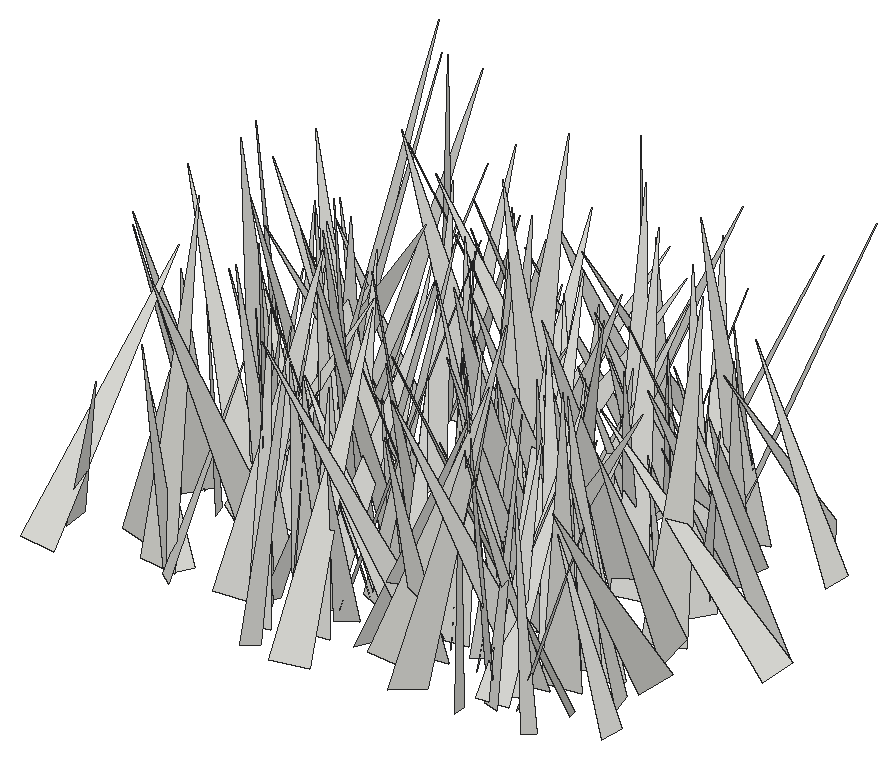
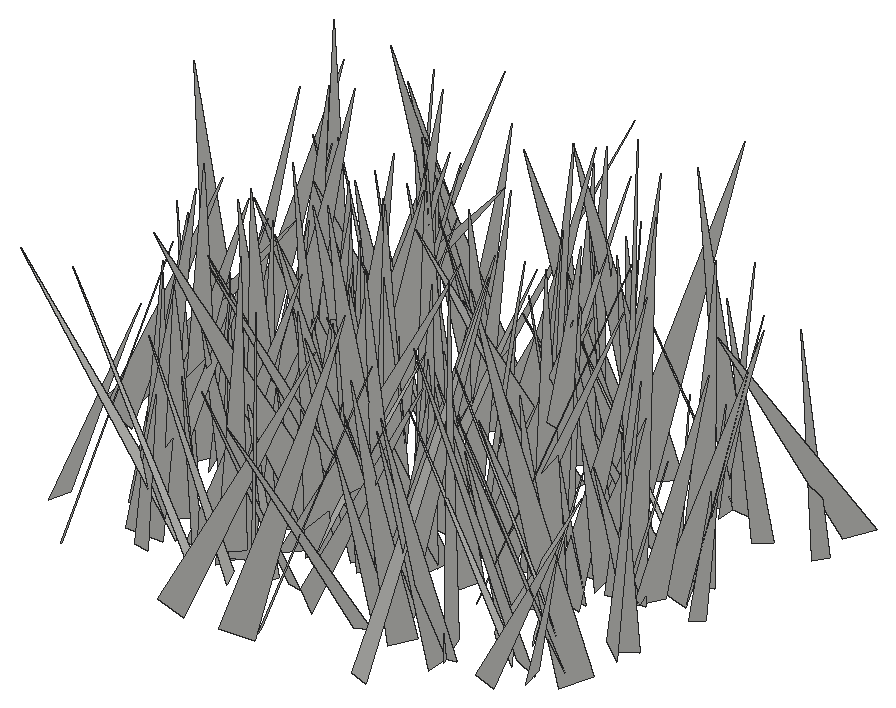
# SketchUp Ruby script. Lengths in inches.
U = 1.inch
M = Sketchup.active_model
def pt(a) = Geom::Point3d.new(a.map { |v| v * U })
def face(e, loops, mat)
  f = e.add_face(loops[0].map { |a| pt(a) })
  loops[1..].each { |l| e.add_face(l.map { |a| pt(a) }).erase! }
  f.material = f.back_material = mat if mat
  f
end
# faces: each face lists its corners as indices into pts; further lists are holes
def faces(e, pts, list, mat = nil) = list.each { |f| face(e, (f[0].is_a?(Array) ? f : [f]).map { |l| l.map { |i| pts[i] } }, mat) }
# xy, xz, yz: faces in a plane at the given z, y or x. An outline is a flat list of corners, or four numbers for a rectangle; further outlines are holes
def ring(l) = l.size == 4 ? [[l[0], l[1]], [l[2], l[1]], [l[2], l[3]], [l[0], l[3]]] : l.each_slice(2).to_a
def flat(e, list, mat, &to3) = list.each { |f| face(e, (f[0].is_a?(Array) ? f : [f]).map { |l| ring(l).map { |u, v| to3.(u, v) } }, mat) }
def xy(e, z, list, mat = nil) = flat(e, list, mat) { |x, y| [x, y, z] }
def xz(e, y, list, mat = nil) = flat(e, list, mat) { |x, z| [x, y, z] }
def yz(e, x, list, mat = nil) = flat(e, list, mat) { |y, z| [x, y, z] }
def lines(e, pts, list) = list.each { |a, b| e.add_line(pt(pts[a]), pt(pts[b])) }
# prism: a flat outline (further loops are holes) pulled along v
def prism(e, loops, v, mat = nil)
  f = face(e, loops, mat); d = Geom::Vector3d.new(v.map { |x| x * U })
  f.pushpull(f.normal.samedirection?(d) ? d.length : -d.length)
end
def box(e, o, s, mat = nil) = prism(e, [[o, [o[0] + s[0], o[1], o[2]], [o[0] + s[0], o[1] + s[1], o[2]], [o[0], o[1] + s[1], o[2]]]], [0, 0, s[2]], mat)
def at(x, y, z, deg = 0) = Geom::Transformation.translation(pt([x, y, z])) * Geom::Transformation.rotation(ORIGIN, Z_AXIS, deg.degrees)
def axes(o, x, y, z) = Geom::Transformation.new([*x, 0, *y, 0, *z, 0, *pt(o).to_a, 1])
def part(name) = M.definitions.add(name)
# library, detail: a bought-in or finely detailed component or shape, given as its bounding box
def library(name, o, s) = part(name).tap { |d| box(d.entities, o, s) }
def detail(e, o, s) = box(e.add_group.entities, o, s)
def put(e, d, t, mat = nil) = e.add_instance(d, t).tap { |i| i.material = mat if mat }
def group(e, t, mat = nil) = e.add_group.tap { |g| g.transformation = t; g.material = mat if mat }.entities
root = M.entities
c1 = part("fur_instance\#9")
p = [[0.8125,0,1.79],[0.67,-0.02,1.48],[0,-0.11,0],[0,0.11,0]]
faces(c1.entities,p,[[0,1,2,3]])
put(root,c1,axes([127.42,270.56,-27.1],[0.8568,-5.86099,0.80486],[-5.91149,-0.87995,-0.11477],[-0.231,0.77949,5.92218]))
put(root,c1,axes([121.75,270.07,-27.1],[1.49133,-6.04191,1.54576],[-6.23212,-1.50337,0.13646],[-0.23383,1.53405,6.22175]))
put(root,c1,axes([127.07,271.05,-27.1],[-7.35388,-1.92649,0.06127],[-1.88282,7.23164,1.39751],[0.41243,-1.33667,7.47248]))
put(root,c1,axes([123.36,266.85,-27.1],[-3.83392,6.10516,1.11787],[5.9137,3.99214,-1.52073],[1.88436,-0.10697,7.04694]))
put(root,c1,axes([114.97,270.12,-27.1],[-4.71927,-1.33587,1.95814],[-1.09743,5.09822,0.83318],[2.10107,-0.33763,4.83341]))
put(root,c1,axes([122.98,270.82,-27.1],[2.32528,-3.90872,0.2043],[-3.90658,-2.33236,-0.15975],[-0.24182,0.09371,4.54527]))
put(root,c1,axes([130.97,271.93,-27.1],[-7.04471,-1.4589,1.32068],[-0.96261,6.83613,2.41686],[1.71638,-2.15394,6.77607]))
put(root,c1,axes([130.64,268.0625,-27.1],[-5.01766,-1.40088,1.70753],[-1.93126,4.83928,-1.7049],[1.07162,2.16194,4.92267]))
put(root,c1,axes([109.97,270.61,-27.1],[4.41728,-0.60705,0.29796],[-0.51929,-4.30631,-1.07505],[-0.43316,-1.02804,4.32726]))
put(root,c1,axes([121.25,267.11,-27.1],[-5.97598,0.81352,1.54005],[0.17172,5.75229,-2.37225],[1.73323,2.235,5.54496]))
put(root,c1,axes([121.75,270.68,-27.1],[4.45698,-3.93649,1.376],[-3.92382,-4.64074,-0.56675],[-1.41173,0.47074,5.91941]))
put(root,c1,axes([128.1,268.14,-27.1],[7.25129,-2.23194,2.73946],[-2.93898,-7.28136,1.84704],[-1.96177,2.6585,7.35875]))
put(root,c1,axes([121.08,269.83,-27.1],[4.15437,2.45212,1.76514],[2.75663,-4.30471,-0.50784],[-1.23677,-1.35794,4.79727]))
put(root,c1,axes([126.07,269.39,-27.1],[3.27115,-5.93629,2.22387],[-6.24966,-2.60094,2.25],[1.06155,2.98013,6.39355]))
put(root,c1,axes([118,272.57,-27.1],[3.07442,-7.15508,0.96712],[-6.88437,-3.22185,-1.95131],[-2.1762,0.08396,7.5392]))
put(root,c1,axes([122.84,269.21,-27.1],[-0.37436,4.96388,1.61425],[5.21969,0.34743,0.14211],[-0.02763,-1.62026,4.97594]))
put(root,c1,axes([132.09,270.02,-27.1],[4.65437,1.55789,0.49043],[1.62302,-4.57734,-0.86283],[-0.1826,-0.97553,4.83174]))
put(root,c1,axes([136.32,270.28,-27.1],[-4.20728,0.83557,0.99678],[1.00115,4.23485,0.67581],[0.83033,-0.87227,4.23588]))
put(root,c1,axes([130.74,269.85,-27.1],[3.92843,5.06138,3.38638],[5.5366,-4.64662,0.52215],[-2.53598,-2.30413,6.38572]))
put(root,c1,axes([120.65,268.35,-27.1],[0.64289,6.12986,1.03372],[6.0316,-0.86662,1.38779],[-1.50455,-0.85491,6.00521]))
put(root,c1,axes([133.84,268.3,-27.1],[-4.92435,-0.05312,0.24709],[-0.15186,4.47527,-2.06445],[0.20202,2.06935,4.47102]))
put(root,c1,axes([119.71,270.26,-27.1],[4.16125,-1.09144,0.28201],[-1.11074,-4.15389,0.31328],[-0.19241,0.37504,4.29058]))
put(root,c1,axes([112.49,270.96,-27.1],[0.76926,-4.66703,1.07076],[-4.59745,-0.41678,1.48633],[1.33832,1.25083,4.49041]))
put(root,c1,axes([126.06,270.8,-27.1],[-4.18794,0.93567,0.33129],[0.9893,4.05153,1.06324],[0.08071,-1.11073,4.15738]))
put(root,c1,axes([124.67,269.99,-27.1],[6.16079,-1.33707,0.34037],[-1.37023,-6.11166,0.79308],[-0.16154,0.84778,6.25413]))
put(root,c1,axes([132.01,271.26,-27.1],[-1.08629,-5.09453,1.21583],[-5.17343,0.84989,-1.06105],[-0.81738,1.39139,5.09985]))
put(root,c1,axes([115.7,270.01,-27.1],[-3.05082,2.35934,0.28628],[2.37608,3.01778,0.45074],[-0.05159,-0.53147,3.83025]))
put(root,c1,axes([114.69,269.6875,-27.1],[0.76042,7.54721,2.45249],[7.93568,-0.724,-0.23253],[-0.00259,-2.46349,7.58186]))
put(root,c1,axes([135.22,274.29,-27.1],[5.40671,-4.03304,0.21931],[-3.53675,-4.90438,-2.9974],[-1.95061,-2.2864,6.04264]))
put(root,c1,axes([119.75,270.36,-27.1],[4.32475,3.25099,2.86901],[3.37923,-5.06616,0.64681],[-2.71679,-1.12634,5.37159]))
put(root,c1,axes([115.56,269.07,-27.1],[2.99735,3.72962,0.28981],[3.68324,-3.00724,0.60693],[-0.65404,0.15682,4.74613]))
put(root,c1,axes([132.59,271.86,-27.1],[2.16747,-6.96935,1.82134],[-7.20329,-2.08612,0.58967],[0.04123,1.91397,7.27476]))
put(root,c1,axes([131.39,269.05,-27.1],[2.56304,5.03632,1.18387],[4.82189,-2.80423,1.49027],[-1.87495,-0.32715,5.45094]))
put(root,c1,axes([118.48,269.61,-27.1],[-2.56408,6.91655,2.55207],[6.94878,3.17004,-1.60986],[2.46298,-1.74312,7.19872]))
put(root,c1,axes([134.1875,270.53,-27.1],[-5.38862,-5.55187,0.24968],[-4.68183,4.34761,-4.37054],[-2.99434,3.19341,6.38427]))
put(root,c1,axes([118.8125,271.9,-27.1],[-6.63003,0.58928,2.6026],[0.94805,7.03587,0.82207],[2.49439,-1.10786,6.6052]))
put(root,c1,axes([131.35,269.95,-27.1],[-4.05743,3.11883,1.27429],[2.94276,4.25195,-1.03673],[1.64046,0.08657,5.0115]))
put(root,c1,axes([110.04,268.16,-27.1],[-2.9172,5.75801,0.16061],[5.28877,2.74872,-2.48273],[2.2824,0.99014,5.95825]))
put(root,c1,axes([126.52,270.12,-27.1],[-2.91757,4.706,0.99504],[4.75363,2.9987,-0.24403],[0.73452,-0.71423,5.53165]))
put(root,c1,axes([129.02,271.27,-27.1],[3.30079,2.00098,0.99665],[2.11543,-3.37049,-0.23912],[-0.72261,-0.72685,3.85253]))
put(root,c1,axes([122.03,273.26,-27.1],[-4.79453,-5.10071,1.01007],[-5.15614,4.84133,-0.02673],[0.67211,0.75447,7.00029]))
put(root,c1,axes([128.05,273.51,-27.1],[5.66121,2.03663,0.41958],[1.99596,-4.98096,-2.75306],[0.58316,-2.72311,5.34956]))
put(root,c1,axes([135.13,272.32,-27.1],[-4.98874,-1.77944,1.14235],[-1.81158,5.1064,0.04294],[1.09068,0.3424,5.29642]))
put(root,c1,axes([131.25,269.32,-27.1],[-3.49002,4.97532,0.38419],[4.70613,3.43753,-1.76559],[1.65943,0.71499,5.81522]))
put(root,c1,axes([116.8,273.88,-27.1],[-4.19902,-6.23031,2.61813],[-6.01537,4.8505,1.89504],[3.08005,0.97931,7.27031]))
put(root,c1,axes([127.11,272.03,-27.1],[-1.46748,5.77462,2.34569],[6.13429,1.76496,-0.50731],[1.10405,-2.13089,5.93652]))
put(root,c1,axes([126.41,272.37,-27.1],[5.41159,0.09186,1.28906],[0.07062,-5.56242,0.09991],[-1.29039,0.08081,5.41145]))
put(root,c1,axes([132.98,273.75,-27.1],[2.11565,-6.08651,1.80009],[-6.2822,-2.27872,-0.32139],[-0.90548,1.58863,6.43571]))
put(root,c1,axes([116.19,273.82,-27.1],[5.48101,-1.25937,0.85366],[-1.15676,-5.52263,-0.72019],[-0.98826,-0.52035,5.57753]))
put(root,c1,axes([116.03,272.39,-27.1],[3.45283,2.51437,0.03768],[2.48973,-3.40925,-0.65094],[0.3531,-0.54815,4.22141]))
put(root,c1,axes([123.1,273.23,-27.1],[-4.21656,2.08304,0.19454],[2.06998,4.09043,1.06765],[-0.30342,-1.04195,4.58024]))
put(root,c1,axes([128.22,275.07,-27.1],[-3.59271,-3.52154,0.36411],[-3.38524,3.56898,1.11534],[1.03633,-0.55007,4.90559]))
put(root,c1,axes([133.88,273.48,-27.1],[1.42768,-3.34431,1.65268],[-3.54003,-1.77266,-0.52903],[-1.17641,1.27565,3.59761]))
put(root,c1,axes([123.36,275.24,-27.1],[-0.67207,-6.04885,0.74296],[-6.03248,0.76649,0.78356],[0.86591,0.6451,6.03542]))
put(root,c1,axes([129.29,274.77,-27.1],[-0.74587,-6.40704,1.23448],[-6.45249,0.53969,-1.09751],[-0.96927,1.33753,6.35625]))
put(root,c1,axes([112.27,275.28,-27.1],[4.76035,-4.27512,0.72339],[-4.20428,-4.81383,-0.78223],[-1.06017,-0.10597,6.35025]))
put(root,c1,axes([134.24,276.65,-27.1],[6.25747,-1.85529,1.59771],[-1.00282,-5.94215,-2.97253],[-2.23363,-2.52972,5.81052]))
put(root,c1,axes([127.14,271.94,-27.1],[5.31118,5.11176,2.74997],[4.78098,-5.96627,1.85658],[-3.29161,-0.41778,7.13385]))
put(root,c1,axes([129.2,273.22,-27.1],[-7.32876,-0.97242,0.83606],[-1.07916,7.29688,-0.97277],[0.69283,1.07947,7.32872]))
put(root,c1,axes([121.81,275.6,-27.1],[-2.25691,-7.5793,1.44794],[-7.71352,2.17504,-0.63772],[-0.20948,1.56823,7.88243]))
put(root,c1,axes([125.21,274.68,-27.1],[-3.55918,-3.90599,0.48478],[-3.91702,3.45103,-0.95229],[-0.38568,0.99656,5.19785]))
put(root,c1,axes([128.62,271.69,-27.1],[1.86893,4.92203,0.04113],[4.36091,-1.67616,2.42774],[-2.28266,0.8277,4.67176]))
put(root,c1,axes([124.77,275.62,-27.1],[4.05285,-0.43746,0.41546],[-0.3233,-3.95717,-1.01285],[-0.50937,-0.96903,3.94856]))
put(root,c1,axes([122.45,274.5,-27.1],[0.90627,3.33198,1.59944],[3.57947,-1.20149,0.47479],[-0.9207,-1.39138,3.42023]))
put(root,c1,axes([112.03,276.02,-27.1],[-5.14482,-3.13912,1.24988],[-3.04737,5.29445,0.7535],[1.4594,-0.01101,5.97959]))
put(root,c1,axes([113.89,274.38,-27.1],[-3.72029,-1.54775,1.40082],[-1.82397,3.80239,-0.64288],[1.01535,1.15959,3.97778]))
put(root,c1,axes([130.78,273.8,-27.1],[-2.14866,5.91991,1.32548],[6.06222,2.04254,0.70466],[-0.22751,-1.48381,6.25824]))
put(root,c1,axes([122.1875,271.52,-27.1],[6.2923,4.31715,0.79405],[3.75537,-6.01297,2.93303],[-2.27277,2.01685,7.04472]))
put(root,c1,axes([118.12,277.77,-27.1],[-1.88375,-7.99896,1.23534],[-7.80751,2.13018,1.88761],[2.13359,0.73274,7.99805]))
put(root,c1,axes([124.57,275.87,-27.1],[4.01557,-5.25956,2.05629],[-5.53772,-4.16187,0.169],[-1.10676,1.74125,6.61508]))
put(root,c1,axes([122.62,272.67,-27.1],[3.92721,6.27569,0.86047],[6.07775,-4.01843,1.56873],[-1.78486,0.12492,7.23508]))
put(root,c1,axes([125.4375,278.36,-27.1],[4.78768,-6.87101,0.53821],[-6.76798,-4.81092,-1.21319],[-1.30189,-0.25808,8.28619]))
put(root,c1,axes([112.44,276.5,-27.1],[-0.64276,-5.9949,1.38637],[-6.03632,0.34404,-1.31091],[-1.1932,1.48889,5.88502]))
put(root,c1,axes([120.71,272.51,-27.1],[-4.56425,4.1816,0.8559],[3.58274,4.43445,-2.55936],[2.31998,1.37862,5.63629]))
put(root,c1,axes([114.54,274.4,-27.1],[2.28513,5.39499,0.34939],[5.12885,-2.04337,-1.99232],[1.70965,-1.08097,5.50984]))
put(root,c1,axes([110.66,277.23,-27.1],[4.01864,-1.00258,0.99057],[-0.63294,-3.95809,-1.43832],[-1.25928,-1.21004,3.88405]))
put(root,c1,axes([119.65,275.46,-27.1],[-6.31517,-2.67121,2.41272],[-3.08957,6.52254,-0.86542],[1.84694,1.77736,6.80204]))
put(root,c1,axes([127.1,275.93,-27.1],[4.74645,-3.63152,0.20608],[-3.44873,-4.38539,2.15263],[1.15614,1.82746,5.57521]))
put(root,c1,axes([119.5,274.42,-27.1],[-6.71,0.21588,0.88951],[-0.0468,6.49159,-1.92847],[0.91413,1.91692,6.43053]))
put(root,c1,axes([116.85,274.99,-27.1],[-1.85743,4.94831,0.92273],[4.99711,1.93095,-0.29602],[0.60509,-0.75691,5.27714]))
put(root,c1,axes([130.01,279.32,-27.1],[2.00321,-7.73932,0.37509],[-7.71802,-2.02729,-0.61059],[-0.68548,0.20889,7.97102]))
put(root,c1,axes([121.49,277.14,-27.1],[1.52564,-3.34819,0.07276],[-3.07421,-1.36842,1.48995],[1.32851,0.67846,3.36423]))
put(root,c1,axes([127.65,276.94,-27.1],[-2.05605,-4.2865,1.82271],[-4.5186,2.31917,0.35698],[1.13077,1.47345,4.74068]))
put(root,c1,axes([113.77,277.75,-27.1],[1.30407,-7.61557,2.3618],[-7.95747,-1.39423,-0.10194],[-0.50366,2.30972,7.72574]))
put(root,c1,axes([133.57,276.84,-27.1],[-3.8242,6.03816,3.67075],[6.53219,4.61268,-0.78232],[2.69524,-2.61192,7.10435]))
put(root,c1,axes([128.375,276.375,-27.1],[2.97809,2.23148,0.68885],[2.24903,-3.04112,0.12836],[-0.62921,-0.30835,3.71915]))
put(root,c1,axes([128.8,274.57,-27.1],[-3.78371,6.02543,0.57396],[5.96039,3.82698,-0.88298],[1.05307,-0.01122,7.05993]))
put(root,c1,axes([138.27,277.92,-27.1],[-5.02457,3.67244,0.21301],[3.24783,4.25941,3.17608],[-1.72736,-2.67378,5.35216]))
put(root,c1,axes([120.51,278.19,-27.1],[-3.95359,-4.39819,1.62013],[-4.4402,4.19331,0.54823],[1.50116,0.81969,5.8885]))
put(root,c1,axes([133.375,277.16,-27.1],[-3.75742,-0.36081,1.22113],[-0.40687,3.94545,-0.08619],[1.20657,0.20686,3.77372]))
put(root,c1,axes([127.06,279.53,-27.1],[1.34944,-6.66989,1.0863],[-6.57389,-1.5523,-1.36482],[-1.56569,0.76902,6.66676]))
put(root,c1,axes([126.93,276.61,-27.1],[-2.07994,4.49979,1.08625],[4.57933,2.1742,-0.23818],[0.67657,-0.88257,4.95151]))
put(root,c1,axes([127.15,279.88,-27.1],[3.45501,-4.88886,0.26504],[-4.85303,-3.46254,-0.60598],[-0.64754,-0.13474,5.95575]))
put(root,c1,axes([112.99,277.23,-27.1],[-5.78073,2.46703,0.60773],[2.49572,5.79658,0.20851],[0.47643,-0.43109,6.28168]))
put(root,c1,axes([120.31,277.21,-27.1],[-1.88222,6.06948,1.49765],[6.0067,1.32242,2.18977],[-1.73238,-2.00921,5.96542]))
put(root,c1,axes([115.4375,279.26,-27.1],[-1.29627,-6.42722,1.30707],[-6.54569,1.18361,-0.67151],[-0.41416,1.4099,6.52216]))
put(root,c1,axes([114.96,278.94,-27.1],[3.94876,4.2171,2.00571],[4.64379,-3.26946,-2.26834],[0.4919,-2.98768,5.31331]))
put(root,c1,axes([118.19,281.13,-27.1],[-6.16351,-3.9605,0.27898],[-3.73191,5.95492,2.08903],[1.35509,-1.6142,7.02213]))
put(root,c1,axes([126.96,279.78,-27.1],[3.0521,-3.8403,0.46149],[-3.78154,-3.08617,-0.67208],[-0.8129,-0.06212,4.85917]))
put(root,c1,axes([115.87,277.18,-27.1],[-2.49681,4.68547,0.3153],[4.52882,2.308,1.56527],[-1.24213,-1.0033,5.07323]))
put(root,c1,axes([137.68,278.66,-27.1],[-0.80032,5.57612,2.90873],[5.9333,-0.30294,2.21326],[-2.08561,-3.00158,5.18026]))
put(root,c1,axes([117.55,278.12,-27.1],[3.71191,-5.65782,4.04126],[-6.28277,-4.69165,-0.79764],[-2.97818,2.84578,6.7196]))
put(root,c1,axes([128.4,277.24,-27.1],[-3.95695,1.67084,0.9926],[1.45221,4.03835,-1.00857],[1.29152,0.5783,4.17516]))
put(root,c1,axes([119.03,278.5625,-27.1],[-7.40149,0.22253,0.007],[0.22253,7.40149,0.00759],[0.00677,-0.0078,7.40483]))
put(root,c1,axes([115.65,280.05,-27.1],[5.14782,-4.26055,1.16689],[-4.27581,-5.25589,-0.32723],[-1.10966,0.4872,6.67423]))
put(root,c1,axes([126.0625,280.6,-27.1],[7.05622,-1.23215,0.51957],[-1.10047,-6.93599,-1.50315],[-0.75967,-1.39725,7.0035]))
put(root,c1,axes([112.97,279.07,-27.1],[-3.79015,-1.11399,0.60809],[-1.15598,3.82064,-0.20588],[0.52388,0.37109,3.9451]))
put(root,c1,axes([132.7,280.36,-27.1],[-1.98967,-4.65459,1.69235],[-4.24096,2.54317,2.00863],[2.55803,0.59592,4.64644]))
put(root,c1,axes([123.68,279.96,-27.1],[0.0585,-4.06465,0.78718],[-4.11626,0.02739,0.44734],[0.44434,0.78888,4.04038]))
put(root,c1,axes([128.87,280.8,-27.1],[-0.89521,-5.51634,1.09126],[-5.41102,1.14576,1.35291],[1.53027,0.82431,5.42227]))
put(root,c1,axes([113.2,278.01,-27.1],[-3.70619,1.07071,1.22273],[0.63141,3.75399,-1.37341],[1.4976,1.06701,3.605]))
put(root,c1,axes([125.53,280.3125,-27.1],[3.59874,-6.83955,3.08177],[-7.12327,-4.18751,-0.97538],[-2.35281,2.21652,7.66674]))
put(root,c1,axes([123.65,279.55,-27.1],[-2.45983,6.23998,3.07468],[6.83629,2.77173,-0.15592],[1.28687,-2.79677,6.7055]))
put(root,c1,axes([111.18,280.77,-27.1],[0.91273,-4.1627,0.50654],[-4.12867,-0.80133,0.85424],[0.734,0.66898,4.1751]))
put(root,c1,axes([115.26,277.03,-27.1],[-5.60466,1.1961,0.32776],[0.92969,5.05609,-2.5538],[0.82084,2.4404,5.13039]))
put(root,c1,axes([122.8125,280.15,-27.1],[7.01983,-0.71592,2.31882],[-0.6287,-7.39114,-0.37866],[-2.34397,-0.1616,7.04608]))
put(root,c1,axes([133.1,282.32,-27.1],[2.61621,-5.42084,0.25429],[-5.22177,-2.59146,-1.52055],[-1.47757,-0.43991,5.82391]))
put(root,c1,axes([134.76,280.34,-27.1],[-1.27388,-3.61865,0.59779],[-3.46584,0.98064,-1.44951],[-1.19998,1.0092,3.55195]))
put(root,c1,axes([122.98,277.87,-27.1],[-0.78819,5.89997,0.04998],[5.7265,0.75282,1.4401],[-1.42105,-0.23877,5.77555]))
put(root,c1,axes([116.57,279.26,-27.1],[-1.7521,4.37342,1.24469],[4.49457,1.86786,-0.23622],[0.6891,-1.06311,4.7054]))
put(root,c1,axes([133.18,279.375,-27.1],[-6.12251,3.37612,2.03098],[3.42132,6.417,-0.35327],[1.95387,-0.65732,6.98272]))
put(root,c1,axes([121.59,280.3,-27.1],[-0.9402,5.50023,2.63792],[6.09336,0.97222,0.14463],[0.28664,-2.62629,5.57814]))
put(root,c1,axes([120.91,280.24,-27.1],[4.20762,-3.32651,0.12048],[-3.15177,-3.91891,1.86887],[1.07075,1.53645,5.02763]))
put(root,c1,axes([127.08,278.2,-27.1],[2.4518,5.85296,0.01413],[5.81055,-2.43218,-0.76857],[0.70347,-0.30989,6.29903]))
put(root,c1,axes([129.95,281.01,-27.1],[-0.88602,-4.48963,1.06047],[-4.46813,0.56653,-1.33464],[-1.14769,1.26043,4.37728]))
put(root,c1,axes([116.01,279.45,-27.1],[4.17653,-0.25853,0.87813],[-0.4857,-4.1025,1.10224],[-0.77592,1.17643,4.03674]))
put(root,c1,axes([132.71,279,-27.1],[-5.22043,-0.84385,1.05571],[-1.17009,4.93002,-1.84535],[0.67639,2.01552,4.95577]))
put(root,c1,axes([130.25,278.84,-27.1],[-1.2461,7.24945,1.28302],[7.36015,1.19663,0.38699],[-0.1701,-1.32928,7.34558]))
put(root,c1,axes([126.83,279.375,-27.1],[-3.66348,3.88372,0.60062],[3.90017,3.69385,-0.09601],[0.48235,-0.37054,5.33808]))
put(root,c1,axes([130.51,280.83,-27.1],[4.15283,1.56186,1.94961],[1.7605,-4.5132,-0.13443],[-1.7723,-0.82343,4.43479]))
put(root,c1,axes([132.78,283.28,-27.1],[4.609,-3.3139,0.05026],[-3.15306,-4.41083,-1.68231],[-1.0211,-1.33793,5.42168]))
put(root,c1,axes([131.3,279.77,-27.1],[-1.57636,3.66287,0.67143],[3.67727,1.64614,-0.34684],[0.58749,-0.47537,3.97256]))
put(root,c1,axes([123.48,281.2,-27.1],[4.4628,-4.8312,0.78242],[-4.8199,-4.15484,1.83716],[0.84924,1.80724,6.31521]))
put(root,c1,axes([124.81,281.22,-27.1],[3.82808,-2.96393,0.87418],[-3.08142,-3.76593,0.72521],[-0.23226,1.11183,4.78677]))
put(root,c1,axes([127.22,281.33,-27.1],[3.70956,-2.15387,1.10856],[-2.28011,-3.78925,0.26761],[-0.81802,0.79458,4.28116]))
put(root,c1,axes([121.86,281.02,-27.1],[-3.05036,2.77962,1.08054],[2.93347,3.07501,0.37088],[0.53722,-1.00823,4.11016]))
put(root,c1,axes([111.72,281.11,-27.1],[-3.6941,-4.73944,2.34113],[-5.23892,3.66336,-0.85037],[0.70493,2.38895,5.94858]))
put(root,c1,axes([131.99,283.66,-27.1],[-3.10911,-5.59083,0.18925],[-5.58666,3.11434,0.22319],[0.28707,0.05678,6.39328]))
put(root,c1,axes([125.95,282.55,-27.1],[-7.5943,2.08618,0.38061],[2.11361,7.33132,1.9887],[-0.17228,-2.01745,7.62041]))
put(root,c1,axes([114.55,282.35,-27.1],[-3.02688,-2.08558,0.64094],[-2.07151,3.09116,0.27563],[0.68504,0.13224,3.66547]))
put(root,c1,axes([111.27,283.84,-27.1],[2.01455,-7.63294,0.11302],[-6.59973,-1.68273,3.99311],[3.83642,1.11337,6.80994]))
put(root,c1,axes([120.86,282.94,-27.1],[-6.83352,3.26319,2.339],[3.80782,6.73136,1.73366],[1.27275,-2.61852,7.37155]))
put(root,c1,axes([128.625,280.88,-27.1],[-5.59489,5.13542,2.2708],[5.22691,5.9344,-0.54239],[2.05147,-1.11455,7.57503]))
put(root,c1,axes([116.65,280.54,-27.1],[5.33264,0.16428,1.51785],[-0.27785,-5.31816,1.55174],[-1.50122,1.56784,5.10452]))
put(root,c1,axes([119.16,280.62,-27.1],[-5.25856,3.05312,1.43062],[2.8843,5.44607,-1.02073],[1.74617,0.1987,5.99435]))
put(root,c1,axes([124.99,282.26,-27.1],[3.66382,-3.28739,1.57998],[-3.52995,-3.75957,0.36325],[-0.918,1.33625,4.90903]))
put(root,c1,axes([127.2,284.36,-27.1],[4.74802,-2.11154,0.82126],[-1.70244,-4.58339,-1.94189],[-1.49491,-1.48682,4.81989]))
put(root,c1,axes([122.82,280.84,-27.1],[1.506,6.6666,0.93752],[6.04421,-0.91584,-3.19677],[2.9648,-1.51928,6.04088]))
put(root,c1,axes([125.47,281.99,-27.1],[-5.46904,-3.01802,0.13387],[-2.92547,5.22183,-1.79189],[-0.75368,1.63119,5.98398]))
put(root,c1,axes([121.11,282.77,-27.1],[0.6303,-6.24139,2.24897],[-6.57772,-0.29373,1.02832],[0.86396,2.31708,6.18828]))
put(root,c1,axes([122.41,281.83,-27.1],[-3.47776,6.78239,3.15196],[7.08859,4.09761,-0.99596],[2.38486,-2.28893,7.55669]))
put(root,c1,axes([128.91,284.55,-27.1],[3.32641,-4.64571,1.36805],[-4.19977,-3.59363,-1.99171],[-2.41165,-0.14974,5.35544]))
put(root,c1,axes([116.39,281.7,-27.1],[-0.0874,4.08723,0.80677],[4.1529,0.14964,-0.30818],[0.33125,-0.79758,4.07653]))
put(root,c1,axes([115.68,283.17,-27.1],[-2.7303,-2.91554,0.15676],[-2.8364,2.59761,-1.08937],[-0.69267,0.85529,3.84294]))
put(root,c1,axes([131.625,283.79,-27.1],[0.51611,-4.80053,1.29544],[-4.96034,-0.40702,0.46794],[0.34389,1.33374,4.80546]))
put(root,c1,axes([123.13,280.91,-27.1],[-3.56356,5.20391,0.71647],[5.00613,3.62664,-1.4419],[1.59144,0.24443,6.14008]))
put(root,c1,axes([125.91,280.6,-27.1],[7.47799,-1.52657,1.95795],[-2.25093,-6.79047,3.30259],[-1.04752,3.69369,6.88067]))
put(root,c1,axes([125.23,284.79,-27.1],[4.19489,0.81761,0.41517],[0.91291,-3.90671,-1.53042],[-0.08632,-1.58339,3.99042]))
put(root,c1,axes([133.32,287.61,-27.1],[-4.76497,-3.93422,0.44703],[-3.2824,4.31602,2.99679],[2.21445,-2.06803,5.40391]))
put(root,c1,axes([127.37,284.6875,-27.1],[5.69628,-2.00129,2.37758],[-1.98509,-6.1627,-0.4314],[-2.39112,0.34864,6.02217]))
put(root,c1,axes([131.26,285.13,-27.1],[0.92373,-7.0899,2.33425],[-7.39568,-1.18748,-0.68009],[-1.00963,2.21177,7.11741]))
put(root,c1,axes([130.72,285.99,-27.1],[-2.364,-4.99525,1.36106],[-4.8414,2.66304,1.36474],[1.83462,0.59091,5.35523]))
put(root,c1,axes([135.64,284.81,-27.1],[-5.10669,0.68056,0.36828],[0.71376,5.09217,0.48729],[0.29888,-0.53268,5.12875]))
put(root,c1,axes([119.1875,283.9,-27.1],[4.30125,1.72732,0.68489],[1.69718,-4.35514,0.32517],[-0.75649,0.05042,4.6237]))
put(root,c1,axes([130.95,283.33,-27.1],[-4.49131,4.50007,0.95246],[4.50728,4.57122,-0.34355],[0.91773,-0.42777,6.34858]))
put(root,c1,axes([113.27,282.15,-27.1],[5.00071,5.94343,0.88428],[5.7504,-5.06729,1.53914],[-1.74336,0.3341,7.61331]))
put(root,c1,axes([123.21,285.32,-27.1],[-3.40667,-4.88664,0.79026],[-4.79108,3.01371,-2.01797],[-1.2447,1.77411,5.60468]))
put(root,c1,axes([116.49,284.91,-27.1],[7.01213,2.59998,3.36264],[2.81322,-7.70163,0.08845],[-3.18638,-1.07803,7.47811]))
put(root,c1,axes([117.9,288.76,-27.1],[-4.53794,-6.8341,0.16977],[-6.57814,4.42074,2.12406],[1.86058,-1.03861,7.92377]))
put(root,c1,axes([129.11,284.55,-27.1],[-3.597,-0.64897,1.74683],[-0.97146,3.89365,-0.55385],[1.59023,0.91068,3.61287]))
put(root,c1,axes([118.375,285.51,-27.1],[4.08731,-3.32744,0.79787],[-3.41978,-4.01464,0.77613],[-0.11643,1.10699,5.21302]))
put(root,c1,axes([114.38,283.85,-27.1],[4.71146,3.59222,0.48874],[3.58656,-4.73541,0.23065],[-0.52868,-0.11206,5.92019]))
put(root,c1,axes([119.79,284.92,-27.1],[-0.91828,3.53646,1.4047],[3.57282,1.29857,-0.93362],[1.30946,-1.06309,3.53244]))
put(root,c1,axes([112.8,284.6,-27.1],[-3.94683,-0.00707,0.27926],[-0.08275,3.80753,-1.07302],[0.26682,1.07619,3.79817]))
put(root,c1,axes([124.25,284.75,-27.1],[2.1149,3.97719,0.39309],[3.90996,-1.96694,-1.13523],[0.82754,-0.87089,4.35914]))
put(root,c1,axes([114.02,285.97,-27.1],[-0.24742,-3.68689,1.2628],[-3.55064,-0.30834,-1.59591],[-1.60648,1.24932,3.33279]))
put(root,c1,axes([113.45,284.17,-27.1],[3.5873,6.66463,1.07182],[6.75002,-3.55215,-0.50434],[-0.05834,-1.18311,7.55193]))
put(root,c1,axes([123.16,288.22,-27.1],[-4.86193,-2.9811,0.43497],[-2.74592,4.72474,1.68858],[1.2394,-1.22654,5.44739]))
put(root,c1,axes([126.58,285.73,-27.1],[4.75078,2.28793,0.55209],[2.32197,-4.75936,-0.25743],[-0.38451,-0.47246,5.26671]))
put(root,c1,axes([116.26,286.04,-27.1],[4.91416,0.05831,0.74386],[0.02898,-4.96646,0.19783],[-0.74558,0.19125,4.91052]))
put(root,c1,axes([123.64,289.03,-27.1],[3.27903,-5.74844,0.73311],[-5.41958,-3.34021,-1.9507],[-2.05188,-0.36394,6.32387]))
put(root,c1,axes([130.66,283.9375,-27.1],[5.97415,4.42308,0.10738],[4.35531,-5.91092,1.16532],[-0.77872,0.87356,7.3414]))
put(root,c1,axes([112.5625,283.23,-27.1],[3.79972,6.90357,0.39781],[6.61789,-3.76205,2.07507],[-2.00527,0.66563,7.60206]))
put(root,c1,axes([126.88,288.97,-27.1],[0.00181,-5.98408,0.19016],[-5.68264,-0.06159,-1.88392],[-1.88493,0.17992,5.67979]))
put(root,c1,axes([116.4,285.52,-27.1],[-0.03084,5.75903,1.17934],[5.85206,0.14189,-0.53988],[0.55736,-1.17118,5.73375]))
put(root,c1,axes([127.26,286.78,-27.1],[5.75926,3.61485,0.22209],[3.58079,-5.62103,-1.36658],[0.54262,-1.27375,6.66098]))
put(root,c1,axes([125.03,286.3125,-27.1],[-5.7993,-3.05465,2.69516],[-3.68736,5.92923,-1.21419],[1.7315,2.39584,6.44116]))
put(root,c1,axes([120.21,285.65,-27.1],[1.05381,5.0713,0.10966],[4.76326,-0.95083,-1.80217],[1.74396,-0.4674,4.856]))
